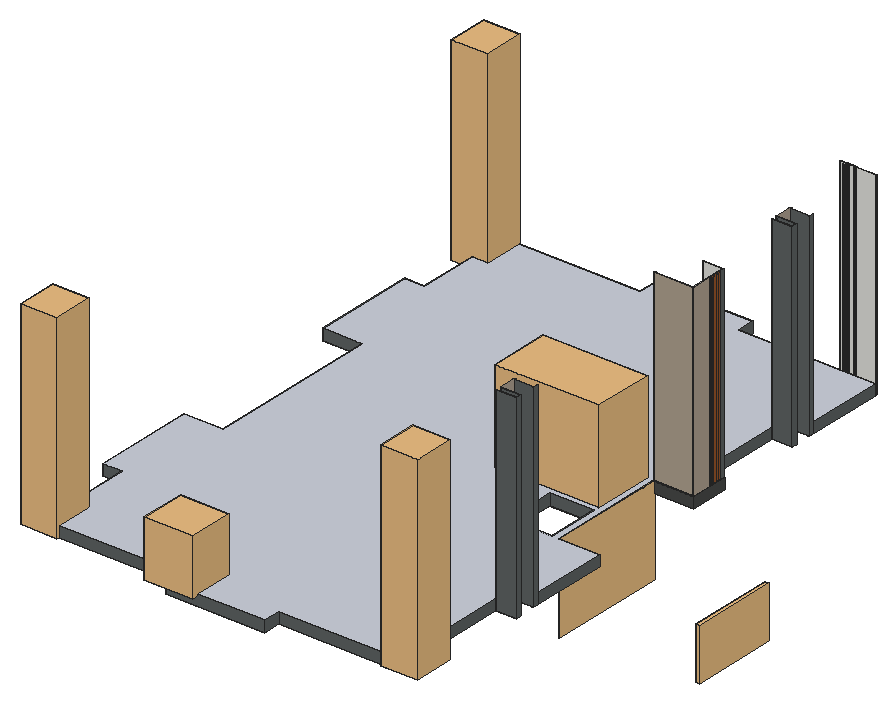
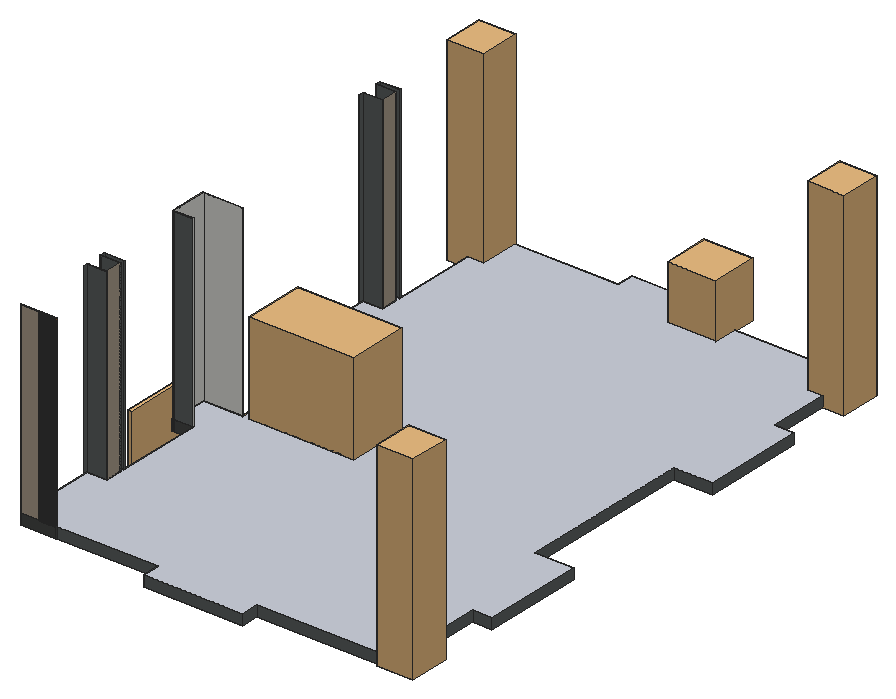
# SketchUp Ruby script. Lengths in inches.
U = 1.inch
M = Sketchup.active_model
def pt(a) = Geom::Point3d.new(a.map { |v| v * U })
def face(e, loops, mat)
  f = e.add_face(loops[0].map { |a| pt(a) })
  loops[1..].each { |l| e.add_face(l.map { |a| pt(a) }).erase! }
  f.material = f.back_material = mat if mat
  f
end
# faces: each face lists its corners as indices into pts; further lists are holes
def faces(e, pts, list, mat = nil) = list.each { |f| face(e, (f[0].is_a?(Array) ? f : [f]).map { |l| l.map { |i| pts[i] } }, mat) }
# xy, xz, yz: faces in a plane at the given z, y or x. An outline is a flat list of corners, or four numbers for a rectangle; further outlines are holes
def ring(l) = l.size == 4 ? [[l[0], l[1]], [l[2], l[1]], [l[2], l[3]], [l[0], l[3]]] : l.each_slice(2).to_a
def flat(e, list, mat, &to3) = list.each { |f| face(e, (f[0].is_a?(Array) ? f : [f]).map { |l| ring(l).map { |u, v| to3.(u, v) } }, mat) }
def xy(e, z, list, mat = nil) = flat(e, list, mat) { |x, y| [x, y, z] }
def xz(e, y, list, mat = nil) = flat(e, list, mat) { |x, z| [x, y, z] }
def yz(e, x, list, mat = nil) = flat(e, list, mat) { |y, z| [x, y, z] }
def lines(e, pts, list) = list.each { |a, b| e.add_line(pt(pts[a]), pt(pts[b])) }
# prism: a flat outline (further loops are holes) pulled along v
def prism(e, loops, v, mat = nil)
  f = face(e, loops, mat); d = Geom::Vector3d.new(v.map { |x| x * U })
  f.pushpull(f.normal.samedirection?(d) ? d.length : -d.length)
end
def box(e, o, s, mat = nil) = prism(e, [[o, [o[0] + s[0], o[1], o[2]], [o[0] + s[0], o[1] + s[1], o[2]], [o[0], o[1] + s[1], o[2]]]], [0, 0, s[2]], mat)
def at(x, y, z, deg = 0) = Geom::Transformation.translation(pt([x, y, z])) * Geom::Transformation.rotation(ORIGIN, Z_AXIS, deg.degrees)
def axes(o, x, y, z) = Geom::Transformation.new([*x, 0, *y, 0, *z, 0, *pt(o).to_a, 1])
def part(name) = M.definitions.add(name)
# library, detail: a bought-in or finely detailed component or shape, given as its bounding box
def library(name, o, s) = part(name).tap { |d| box(d.entities, o, s) }
def detail(e, o, s) = box(e.add_group.entities, o, s)
def put(e, d, t, mat = nil) = e.add_instance(d, t).tap { |i| i.material = mat if mat }
def group(e, t, mat = nil) = e.add_group.tap { |g| g.transformation = t; g.material = mat if mat }.entities
root = M.entities
M.materials.add("1487 AP 8286 CHARCOAL SHADOW").color = [94, 99, 99]
M.materials.add("1488 AP 8285 MINESHAFT").color = [72, 74, 72]
M.materials.add("W149Z659F75_NILAYA ARCHITECTURE FD25355 ROLL F1").color = [175, 162, 145]
M.materials.add("W149Z659F75_NILAYA ARCHITECTURE FD25355 ROLL F75").color = [176, 162, 144]
M.materials.add("[Marble Carrara Floor Tile]").color = [204, 208, 219]
M.materials.add("[Wood Cherry Original]").color = [152, 86, 42]
c1 = library("Gate_Lasercut_10ftx6ft_Kalil",[-0.15,-3.25,-0.15],[120,5.625,60.3])
c2 = library("Group\#130",[0,6,-42],[1.25,152,114])
c3 = part("Group247\#1")
box(c3.entities,[-12,-129,0],[2,258,0.5])
c4 = part("Group248\#1")
box(c4.entities,[-9.5,-129,0],[2,258,0.5])
c5 = part("Group249\#1")
box(c5.entities,[-7,-129,0],[2,258,0.5])
c6 = part("Group250\#1")
box(c6.entities,[-4.5,-129,0],[2,258,0.5])
c7 = part("Group251\#1")
box(c7.entities,[-2,-129,0],[2,258,0.5])
c8 = part("Group252\#1")
box(c8.entities,[0.5,-129,0],[2,258,0.5])
c9 = part("Group253\#1")
box(c9.entities,[3,-129,0],[2,258,0.5])
c10 = part("Group254\#1")
box(c10.entities,[5.5,-129,0],[2,258,0.5])
c11 = part("Group255\#1")
box(c11.entities,[8,-129,0],[2,258,0.5])
c12 = part("Group256\#1")
box(c12.entities,[10.5,-129,0],[2,258,0.5])
c13 = part("Group245\#1")
put(c13.entities,c3,at(0,0,0))
put(c13.entities,c4,at(0,0,0))
put(c13.entities,c5,at(0,0,0))
put(c13.entities,c6,at(0,0,0))
put(c13.entities,c7,at(0,0,0))
put(c13.entities,c8,at(0,0,0))
put(c13.entities,c9,at(0,0,0))
put(c13.entities,c10,at(0,0,0))
put(c13.entities,c11,at(0,0,0))
put(c13.entities,c12,at(0,0,0))
c14 = part("Group220\#1")
box(c14.entities,[-9.875,-130.5,0],[2,261,0.5])
c15 = part("Group221\#1")
box(c15.entities,[-7.375,-130.5,0],[2,261,0.5])
c16 = part("Group222\#1")
box(c16.entities,[-4.875,-130.5,0],[2,261,0.5])
c17 = part("Group223\#1")
box(c17.entities,[-2.375,-130.5,0],[2,261,0.5])
c18 = part("Group224\#1")
box(c18.entities,[0.125,-130.5,0],[2,261,0.5])
c19 = part("Group225\#1")
box(c19.entities,[2.625,-130.5,0],[2,261,0.5])
c20 = part("Group226\#1")
box(c20.entities,[5.125,-130.5,0],[2,261,0.5])
c21 = part("Group227\#1")
box(c21.entities,[7.625,-130.5,0],[2,261,0.5])
c22 = part("Group218\#1")
put(c22.entities,c14,at(0,0,0))
put(c22.entities,c15,at(0,0,0))
put(c22.entities,c16,at(0,0,0))
put(c22.entities,c17,at(0,0,0))
put(c22.entities,c18,at(0,0,0))
put(c22.entities,c19,at(0,0,0))
put(c22.entities,c20,at(0,0,0))
put(c22.entities,c21,at(0,0,0))
c23 = part("12")
xy(c23.entities,0,[[-27,-1.5,-27,0.5,27,0.5,27,51,0,51,0,52.25,29.24,52.25,29.24,-1.5]],"1488 AP 8285 MINESHAFT")
xy(c23.entities,12,[[27.49,25.75,28.24,45.5]])
xy(c23.entities,15,[[-27,-1.5,29.24,-1.5,29.24,52.25,0,52.25,0,52,27.99,52,27.99,45.5,28.24,45.5,28.24,-0.5,-27,-0.5]],"1488 AP 8285 MINESHAFT")
xy(c23.entities,273,[[-27,-0.5,28.24,-0.5,28.24,25.75,27,25.75,27,0.5,-27,0.5],[27,25.75,27.49,45.5],[27,45.5,27.99,45.5,27.99,52,0,52,0,51,27,51]])
xz(c23.entities,-1.5,[[-27,0,29.24,15]],"1488 AP 8285 MINESHAFT")
xz(c23.entities,-0.5,[[-27,15,28.24,273]],"W149Z659F75_NILAYA ARCHITECTURE FD25355 ROLL F75")
xz(c23.entities,0.5,[[-27,0,27,273]])
xz(c23.entities,25.75,[[27.49,12,28.24,273]])
xz(c23.entities,45.5,[[27.49,12,27.99,273],[27.99,12,28.24,15]])
xz(c23.entities,51,[[0,0,27,273]])
xz(c23.entities,52,[[0,15,27.99,273]],"1487 AP 8286 CHARCOAL SHADOW")
xz(c23.entities,52.25,[[0,0,29.24,15]],"1488 AP 8285 MINESHAFT")
yz(c23.entities,-27,[[-1.5,0,-1.5,15,-0.5,15,-0.5,273,0.5,273,0.5,0]])
yz(c23.entities,0,[[51,0,51,273,52,273,52,15,52.25,15,52.25,0]])
yz(c23.entities,27,[[0.5,0,51,273]])
yz(c23.entities,27.99,[[45.5,15,52,273]],"1487 AP 8286 CHARCOAL SHADOW")
yz(c23.entities,28.24,[[25.75,12,45.5,15]])
yz(c23.entities,28.24,[[-0.5,15,25.75,273]],"W149Z659F75_NILAYA ARCHITECTURE FD25355 ROLL F75")
yz(c23.entities,29.24,[[-1.5,0,52.25,15]],"1488 AP 8285 MINESHAFT")
put(c23.entities,c22,axes([27.49,35.75,142.5],[0,1,0],[0,0,1],[1,0,0]),"[Wood Cherry Original]")
c24 = part("13")
prism(c24.entities,[[[0,0,-279],[0,1,-279],[28,1,-279],[28,-7,-279],[0,-7,-279],[0,-6,-279],[27,-6,-279],[27,0,-279]]],[0,0,273])
c25 = library("18",[5.5,-2,0],[50.74,55.75,273])
c26 = part("16")
prism(c26.entities,[[[0,0.5,-15],[0,1,-15],[27,1,-15],[27,7,-15],[27.25,7,-15],[27.25,0.5,-15]]],[0,0,273])
c27 = part("Group\#97")
box(c27.entities,[0,0,-15.09],[0.5,22.47,273])
c28 = library("Group\#67",[-15,0,-4],[144,84,130])
c29 = library("Flora+17",[-57.52,158.6,-38.64],[66.99,62.88,77.28])
put(root,c1,axes([801.27,821.39,0.1],[0,-1,0],[1,0,0],[0,0,1.19527]))
put(root,c2,axes([631.5,666.5,54.32],[1,0,0],[0,1.07895,0],[0,0,1.07895]))
g1 = group(root,at(144,357.97,138),"1487 AP 8286 CHARCOAL SHADOW")
xy(g1,-21,[[[216,-24,216,0,0,0,0,51,27,51,27,136.5,0,136.5,0,277.5,54,277.5,54,517.5,0,517.5,0,658.5,27,658.5,27,744,0,744,0,795,216,795,216,819,352.5,819,352.5,795,541.5,795,541.5,681,514.5,681,514.5,657.03,541.5,657.03,541.5,651.03,514.5,651.03,514.5,531,541.5,531,541.5,480,487.5,480,487.5,315,544.5,315,544.5,201,517.5,201,517.5,177.03,544.5,177.03,544.5,171.03,517.5,171.03,517.5,51,544.5,51,544.5,0,352.5,0,352.5,-24],[349.5,396,478.5,480],[418.5,315,478.5,387]]])
xy(g1,-6,[[[216,-24,352.5,-24,352.5,0,544.5,0,544.5,51,517.5,51,517.5,171.03,544.5,171.03,544.5,177.03,517.5,177.03,517.5,201,544.5,201,544.5,315,487.5,315,487.5,480,541.5,480,541.5,531,514.5,531,514.5,651.03,541.5,651.03,541.5,657.03,514.5,657.03,514.5,681,541.5,681,541.5,795,352.5,795,352.5,819,216,819,216,795,0,795,0,744,27,744,27,658.5,0,658.5,0,517.5,54,517.5,54,277.5,0,277.5,0,136.5,27,136.5,27,51,0,51,0,0,216,0],[349.5,396,478.5,480],[418.5,315,478.5,387]]],"[Marble Carrara Floor Tile]")
xz(g1,-24,[[216,-21,352.5,-6]])
xz(g1,0,[[0,-21,216,-6],[352.5,-21,544.5,-6]])
xz(g1,51,[[0,-21,27,-6],[517.5,-21,544.5,-6]])
xz(g1,136.5,[[0,-21,27,-6]])
xz(g1,171.03,[[517.5,-21,544.5,-6]])
xz(g1,177.03,[[517.5,-21,544.5,-6]])
xz(g1,201,[[517.5,-21,544.5,-6]])
xz(g1,277.5,[[0,-21,54,-6]])
xz(g1,315,[[418.5,-21,478.5,-6],[487.5,-21,544.5,-6]])
xz(g1,387,[[418.5,-21,478.5,-6]])
xz(g1,396,[[349.5,-21,478.5,-6]])
xz(g1,480,[[349.5,-21,478.5,-6],[487.5,-21,541.5,-6]])
xz(g1,517.5,[[0,-21,54,-6]])
xz(g1,531,[[514.5,-21,541.5,-6]])
xz(g1,651.03,[[514.5,-21,541.5,-6]])
xz(g1,657.03,[[514.5,-21,541.5,-6]])
xz(g1,658.5,[[0,-21,27,-6]])
xz(g1,681,[[514.5,-21,541.5,-6]])
xz(g1,744,[[0,-21,27,-6]])
xz(g1,795,[[0,-21,216,-6],[352.5,-21,541.5,-6]])
xz(g1,819,[[216,-21,352.5,-6]])
yz(g1,0,[[0,-21,51,-6],[136.5,-21,277.5,-6],[517.5,-21,658.5,-6],[744,-21,795,-6]])
yz(g1,27,[[51,-21,136.5,-6],[658.5,-21,744,-6]])
yz(g1,54,[[277.5,-21,517.5,-6]])
yz(g1,216,[[-24,-21,0,-6],[795,-21,819,-6]])
yz(g1,349.5,[[396,-21,480,-6]])
yz(g1,352.5,[[-24,-21,0,-6],[795,-21,819,-6]])
yz(g1,418.5,[[315,-21,387,-6]])
yz(g1,478.5,[[315,-21,387,-6],[396,-21,480,-6]])
yz(g1,487.5,[[315,-21,480,-6]])
yz(g1,514.5,[[531,-21,651.03,-6],[657.03,-21,681,-6]])
yz(g1,517.5,[[51,-21,171.03,-6],[177.03,-21,201,-6]])
yz(g1,541.5,[[480,-21,531,-6],[651.03,-21,657.03,-6],[681,-21,795,-6]])
yz(g1,544.5,[[0,-21,51,-6],[171.03,-21,177.03,-6],[201,-21,315,-6]])
g2 = group(root,at(635.76,1100.72,117))
xy(g2,0,[[0,52.25,49.74,53.75]],"1488 AP 8285 MINESHAFT")
xy(g2,15,[[0,53.25,24.5,53.75]],"W149Z659F75_NILAYA ARCHITECTURE FD25355 ROLL F75")
xy(g2,273,[[0,52.25,49.74,52.25,49.74,53.75,24.5,53.75,24.5,53.25,0,53.25]])
xz(g2,52.25,[[0,0,49.74,273]])
xz(g2,53.75,[[0,0,49.74,15]],"1488 AP 8285 MINESHAFT")
xz(g2,53.75,[[24.5,15,49.74,273]],"W149Z659F75_NILAYA ARCHITECTURE FD25355 ROLL F75")
yz(g2,0,[[52.25,0,52.25,273,53.25,273,53.25,15,53.75,15,53.75,0]],"1488 AP 8285 MINESHAFT")
yz(g2,24.5,[[53.25,15,53.75,273]],"W149Z659F75_NILAYA ARCHITECTURE FD25355 ROLL F75")
yz(g2,49.74,[[52.25,0,53.75,0,53.75,15,53.25,15,53.25,273,52.25,273]],"1488 AP 8285 MINESHAFT")
yz(g2,49.74,[[53.25,15,53.75,273]],"W149Z659F75_NILAYA ARCHITECTURE FD25355 ROLL F1")
put(g2,c13,axes([12.5,53.25,144],[-1,0,0],[0,0,1],[0,1,0]),"[Wood Cherry Original]")
put(root,c23,at(658.5,837.47,117))
put(root,c24,at(661.5,535,396),"1487 AP 8286 CHARCOAL SHADOW")
put(root,c24,at(658.5,1015,396),"1487 AP 8286 CHARCOAL SHADOW")
put(root,c25,at(634.5,357.47,117))
put(root,c25,axes([198,357.47,117],[-1,0,0],[0,1,0],[0,0,1]))
put(root,c25,at(198,1153.47,117,180))
put(root,c26,at(661.5,557.97,132),"1487 AP 8286 CHARCOAL SHADOW")
put(root,c26,at(658.5,1037.97,132),"1487 AP 8286 CHARCOAL SHADOW")
put(root,c27,at(661.5,536,132.09),"W149Z659F75_NILAYA ARCHITECTURE FD25355 ROLL F1")
put(root,c27,at(658.5,1016,132.09),"W149Z659F75_NILAYA ARCHITECTURE FD25355 ROLL F1")
put(root,c28,at(493.5,753.97,132))
put(root,c29,at(393.59,167.58,168))
